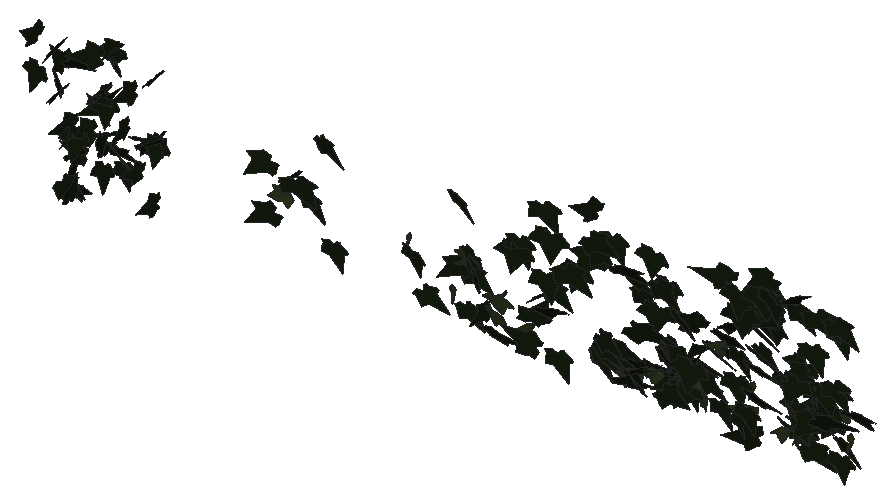
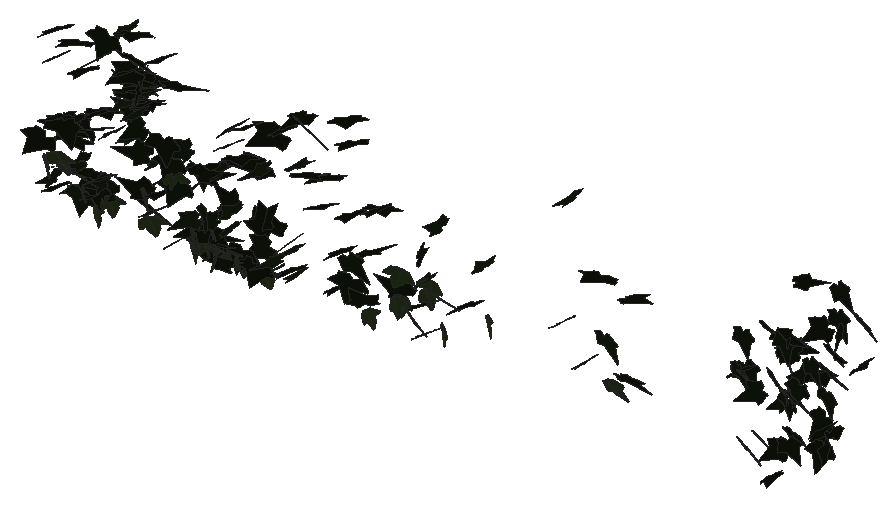
# SketchUp Ruby script. Lengths in millimetres.
U = 1.mm
M = Sketchup.active_model
def pt(a) = Geom::Point3d.new(a.map { |v| v * U })
def face(e, loops, mat)
  f = e.add_face(loops[0].map { |a| pt(a) })
  loops[1..].each { |l| e.add_face(l.map { |a| pt(a) }).erase! }
  f.material = f.back_material = mat if mat
  f
end
# faces: each face lists its corners as indices into pts; further lists are holes
def faces(e, pts, list, mat = nil) = list.each { |f| face(e, (f[0].is_a?(Array) ? f : [f]).map { |l| l.map { |i| pts[i] } }, mat) }
# xy, xz, yz: faces in a plane at the given z, y or x. An outline is a flat list of corners, or four numbers for a rectangle; further outlines are holes
def ring(l) = l.size == 4 ? [[l[0], l[1]], [l[2], l[1]], [l[2], l[3]], [l[0], l[3]]] : l.each_slice(2).to_a
def flat(e, list, mat, &to3) = list.each { |f| face(e, (f[0].is_a?(Array) ? f : [f]).map { |l| ring(l).map { |u, v| to3.(u, v) } }, mat) }
def xy(e, z, list, mat = nil) = flat(e, list, mat) { |x, y| [x, y, z] }
def xz(e, y, list, mat = nil) = flat(e, list, mat) { |x, z| [x, y, z] }
def yz(e, x, list, mat = nil) = flat(e, list, mat) { |y, z| [x, y, z] }
def lines(e, pts, list) = list.each { |a, b| e.add_line(pt(pts[a]), pt(pts[b])) }
# prism: a flat outline (further loops are holes) pulled along v
def prism(e, loops, v, mat = nil)
  f = face(e, loops, mat); d = Geom::Vector3d.new(v.map { |x| x * U })
  f.pushpull(f.normal.samedirection?(d) ? d.length : -d.length)
end
def box(e, o, s, mat = nil) = prism(e, [[o, [o[0] + s[0], o[1], o[2]], [o[0] + s[0], o[1] + s[1], o[2]], [o[0], o[1] + s[1], o[2]]]], [0, 0, s[2]], mat)
def at(x, y, z, deg = 0) = Geom::Transformation.translation(pt([x, y, z])) * Geom::Transformation.rotation(ORIGIN, Z_AXIS, deg.degrees)
def axes(o, x, y, z) = Geom::Transformation.new([*x, 0, *y, 0, *z, 0, *pt(o).to_a, 1])
def part(name) = M.definitions.add(name)
# library, detail: a bought-in or finely detailed component or shape, given as its bounding box
def library(name, o, s) = part(name).tap { |d| box(d.entities, o, s) }
def detail(e, o, s) = box(e.add_group.entities, o, s)
def put(e, d, t, mat = nil) = e.add_instance(d, t).tap { |i| i.material = mat if mat }
def group(e, t, mat = nil) = e.add_group.tap { |g| g.transformation = t; g.material = mat if mat }.entities
root = M.entities
M.materials.add("efeu1").color = [18, 25, 13]
M.materials.add("efeu2").color = [43, 57, 29]
c1 = part("ivyleaf_9")
p = [[39.1,54.8,31.7],[34.5,51.8,30.2],[-5.3,25.2,17.3],[-17.9,28.3,20.9],[-21.6,21.7,17],[-20.2,4.3,5.3],
  [-22.9,-0.3,2.5],[-17.1,-4,-0.6],[-2,-2.1,-1.2],[-0.7,-15.4,-10.1],[16.6,-22.3,-16.7],[21.1,-15.1,-12.5],
  [32.7,-10.7,-11],[46.1,-1.8,-6.6],[30.8,11.2,3.8]]
faces(c1.entities,p,[[0,1,2,3,4,5,6,7,8,9,10,11,12,13,14]],"efeu1")
c2 = part("ivyleaf_10")
p = [[0,12.8,-0.8],[-1.5,51.3,-10.9],[-4.9,51,-11.6],[-13.6,26.5,-7.3],[-13.2,15.9,-4.6],[-21.1,19.3,-7.2],
  [-29.5,16.3,-8.3],[-29.2,8.3,-6.2],[-19.7,-9.8,0.5],[-7.6,-13,4],[1,-12.2,5.8],[-0.4,51.1,-11.1],
  [-1.5,51.1,-10.9],[1,-12.4,5.9],[16.9,-12.4,3.5],[35.1,9.1,-5.1],[35,12.9,-6.1],[20.5,16.4,-4.9],
  [15.8,15,-3.8],[15.3,27.6,-7.1],[12.8,31.3,-7.8]]
faces(c2.entities,p,[[0,1,2,3,4,5,6,7,8,9,10],[11,12,0,13,14,15,16,17,18,19,20]],"efeu2")
put(root,c1,axes([273.7,428,4835.9],[-0.85557,1.08423,0.7221],[-0.62176,0.52637,-1.2853],[-1.46259,-0.858,0.12399]))
put(root,c1,axes([242.2,477.1,4657.7],[-0.36532,-1.32775,0.51119],[-0.11906,-0.50199,-1.36102],[1.73167,-0.31462,0.01427]))
put(root,c1,axes([344.8,510.7,4693.1],[-0.22209,0.63679,1.31638],[-1.04668,1.02774,-0.6158],[-1.44472,-0.84247,0.24378]))
put(root,c1,axes([363.4,626.9,4702.8],[-0.59674,1.20004,-0.36765],[0.22479,-0.32165,-1.29503],[-1.51462,-0.52054,-0.04735]))
put(root,c1,axes([400.9,482.9,4216.3],[-0.00561,-0.17837,1.46528],[0.54141,1.39734,0.1715],[-1.71753,0.44106,0.04927]))
put(root,c1,axes([416.8,537.6,4311.3],[-0.27197,-1.32039,-0.3434],[0.05862,-0.35533,1.33509],[-1.66342,0.20336,0.10319]))
put(root,c1,axes([417.6,371.5,4715.4],[1.01386,-0.28067,-1.21153],[-1.35322,0.49166,-0.87473],[0.68611,1.38445,0.06503]))
put(root,c1,axes([434,676.2,4345.7],[-0.07377,1.1603,-0.56671],[-0.42955,-0.56065,-1.11032],[-1.51569,0.10242,0.34225]))
put(root,c1,axes([444.1,651,4544.6],[-1.33415,0.72884,-0.16345],[0.03182,-0.25235,-1.29979],[-0.91072,-1.07653,0.19402]))
put(root,c1,axes([444.3,349,4884.6],[-0.77185,1.1754,-0.62675],[0.27427,-0.58968,-1.33281],[-1.6018,-0.66735,0.07379]))
put(root,c1,axes([449.2,419.2,4440.2],[-0.37174,1.34751,0.43821],[-0.16281,0.41894,-1.38106],[-1.72103,-0.33069,0.03599]))
put(root,c1,axes([439.7,599.8,4557.9],[0.36998,1.23705,0.48871],[0.02532,0.49679,-1.27039],[-1.62251,0.28984,0.09162]))
put(root,c1,axes([432.2,454,4354.7],[0.66994,1.15124,0.63986],[0.34349,0.57463,-1.27548],[-1.56973,0.61707,-0.00601]))
put(root,c1,axes([425.4,452.9,4758.8],[1.51954,0.5727,0.5016],[0.50025,0.30572,-1.36723],[-0.78257,1.30747,0.09999]))
put(root,c1,axes([444.9,446.4,4213.9],[1.38274,0.72856,-0.4687],[-0.50813,-0.2185,-1.3468],[-0.92673,1.20687,0.03911]))
put(root,c1,axes([489.3,388.7,4527.7],[-1.64876,0.54253,0.34301],[-0.3881,0.12828,-1.45628],[-0.68013,-1.38838,-0.00051]))
put(root,c1,axes([453.5,376.3,4266.3],[0.22516,-0.60274,-1.36473],[-0.17497,1.3616,-0.62075],[1.81169,0.20641,0.10966]))
put(root,c1,axes([495.8,290.9,4720.2],[-0.46741,1.43362,-0.19459],[0.0618,-0.18788,-1.48393],[-1.76397,-0.38646,-0.00043]))
put(root,c1,axes([500.2,620.9,4759.3],[-0.16396,1.3952,-0.04116],[0.01199,-0.04041,-1.40165],[-1.70285,-0.13462,-0.00591]))
put(root,c1,axes([518.3,627.4,4773.2],[-0.26754,-0.15658,-1.36819],[-1.011,-1.09151,0.25774],[-1.34185,0.8536,0.07861]))
put(root,c1,axes([481,720.5,4195.6],[-0.00928,-1.24236,-0.31069],[-0.02096,0.31077,-1.24224],[1.56221,-0.00321,-0.01851]))
put(root,c1,axes([476.1,660.7,4295.4],[1.54093,0.22876,0.34521],[0.41801,0.04508,-1.28351],[-0.28378,1.30861,-0.01613]))
put(root,c1,axes([510.5,630,4681.9],[0.63604,-0.86623,0.94791],[-0.39628,0.90082,1.00185],[-1.51564,-0.59905,0.13585]))
put(root,c1,axes([471.6,540.1,4561],[1.02764,-1.06892,0.55335],[0.42029,-0.43303,-1.36092],[1.40703,0.91005,0.00238]))
put(root,c1,axes([515.7,335.3,4238.7],[-1.21926,0.98729,-0.32059],[-0.33495,0.17776,1.40332],[1.2213,1.03439,0.06482]))
put(root,c1,axes([509.8,391.2,4490.1],[-0.88902,-1.23215,-0.15341],[0.10673,0.12649,-1.43147],[1.51107,-0.73386,0.01085]))
put(root,c1,axes([538.2,445,4496.1],[-0.7733,-0.52593,1.13026],[-0.94644,-0.82614,-0.81947],[1.19053,-0.99837,0.08269]))
put(root,c1,axes([527.9,532.6,4288],[-1.13407,-0.39054,-0.96094],[1.17597,0.15142,-0.99397],[0.46746,-1.32837,0.16922]))
put(root,c1,axes([577.8,501.9,4403.9],[-0.15807,1.16395,0.73041],[-0.26338,0.7073,-1.16542],[-1.65564,-0.22364,0.11566]))
put(root,c1,axes([556.5,471.2,4609.3],[0.39568,0.02009,1.35724],[1.1048,1.03631,-0.23174],[-1.23362,0.93454,0.2278]))
put(root,c1,axes([590.4,461.5,4622.3],[-0.22109,-0.22106,-1.38757],[-0.25021,-1.37992,0.24662],[-1.69582,0.23242,0.14451]))
put(root,c1,axes([606.2,393,4870.9],[-1.02417,-0.18439,1.19989],[-1.38465,-0.39852,-0.85529],[0.52561,-1.40913,0.08488]))
put(root,c1,axes([571.2,448.3,4425.1],[-0.38138,0.87701,1.11033],[0.28619,-1.08925,0.9264],[1.70231,0.3796,0.09301]))
put(root,c1,axes([590.4,468.8,4629.9],[-0.51102,-1.33372,-0.2241],[0.07927,0.21449,-1.39795],[1.64804,-0.42387,-0.00225]))
put(root,c1,axes([577.9,514.2,4410.2],[1.37084,-0.80195,0.15563],[0.15018,-0.09543,-1.38045],[0.98526,1.13034,-0.00613]))
put(root,c1,axes([642.8,610.2,4272],[-1.28412,0.74505,0.34822],[-0.38587,0.15534,-1.28843],[-0.92616,-1.09772,0.05401]))
put(root,c1,axes([639.9,529.9,4511.9],[-1.43164,0.62304,-0.40212],[0.43304,-0.18896,-1.32862],[-0.79429,-1.22599,0.00043]))
put(root,c1,axes([694.9,500.9,4698.8],[-1.57968,0.49729,0.16789],[-0.18829,0.06643,-1.38701],[-0.61203,-1.30396,-0.00663]))
put(root,c1,axes([655.5,574.9,4448],[1.57565,0.15252,0.42652],[0.42907,0.47451,-1.23465],[-0.34826,1.27467,0.40858]))
put(root,c1,axes([702.8,620.3,4710.5],[-0.21174,1.39179,0.02506],[-0.00306,0.02494,-1.40256],[-1.69825,-0.17357,-0.00059]))
put(root,c1,axes([751.8,571.9,4188.3],[-1.51029,0.77954,0.0722],[-0.07438,0.03866,-1.46294],[-0.95221,-1.23944,-0.00023]))
put(root,c1,axes([778.7,516,4492.7],[-0.08106,1.4185,-0.5317],[-0.25474,-0.53571,-1.4031],[-1.83051,0.01173,0.21881]))
put(root,c1,axes([796.7,542.8,4462.4],[-1.30491,0.60869,0.83669],[-0.91036,0.37983,-1.23024],[-0.87444,-1.30377,0.03221]))
put(root,c1,axes([785.8,541.7,4496.2],[-0.6554,1.35212,0.05077],[-0.0876,0.02606,-1.45382],[-1.64843,-0.53898,0.05707]))
put(root,c1,axes([783.9,547.8,4481.5],[-0.55833,-1.36902,0.17153],[0.10373,-0.20836,-1.43612],[1.68007,-0.4421,0.14567]))
put(root,c2,axes([1267.7,738.1,4337.1],[1.34868,-0.41175,-0.9334],[-1.5314,0.47307,-0.81957],[1.19359,1.0722,0.00316]))
put(root,c1,axes([1288.4,631,4313.5],[-2.34815,-0.0339,0.16638],[-0.31584,-0.01743,-1.23419],[0.06836,-1.24484,0.01275]))
put(root,c1,axes([1343.3,535,4603.3],[-1.56454,-0.78213,0.61308],[-0.87792,-0.40443,-1.13447],[1.67525,-0.94238,-0.02196]))
put(root,c1,axes([1359.5,658.4,4477.6],[-0.53506,1.23747,0.10978],[-0.05103,0.10649,-1.269],[-2.36385,-0.2824,0.00255]))
put(root,c1,axes([1402.1,715.4,4382],[0.70204,-1.16725,-0.24276],[-0.05097,0.24593,-1.22322],[2.26848,0.36676,0.04764]))
put(root,c1,axes([1535.1,468.5,4608.6],[-0.5958,-0.87829,-0.93817],[1.31742,0.69832,-0.88473],[2.06074,-0.70037,0.29436]))
put(root,c1,axes([1694.3,504,4363.7],[0.11029,-1.29748,-0.05119],[-0.00218,0.05119,-1.29877],[2.47128,0.05795,0.00114]))
put(root,c1,axes([1709.9,414.3,4874.7],[1.23856,-1.15916,-0.29844],[-0.17967,0.28894,-1.32809],[2.27097,0.65505,0.05769]))
put(root,c2,axes([1908.5,702.4,4378.1],[0.64723,-1.18371,-0.29161],[-0.00315,0.30229,-1.22901],[2.32019,0.33061,0.07968]))
put(root,c1,axes([2086.6,504.3,4469.2],[0.19322,-1.20535,0.54246],[0.18761,-0.53564,-1.20865],[2.50863,0.13289,0.04861]))
put(root,c2,axes([2152.3,675.9,4243.2],[1.0391,-1.09409,-0.25622],[0.18731,0.33033,-1.20082],[2.13038,0.5046,0.23055]))
put(root,c1,axes([2127.5,527.8,4302],[0.86069,-0.89994,-0.83525],[0.00521,0.89084,-0.95835],[2.33677,0.32948,0.30978]))
put(root,c1,axes([2197.1,678.1,4378.7],[-2.3902,0.06796,-0.12555],[0.19895,-0.31928,-1.21851],[-0.18504,-1.22109,0.31161]))
put(root,c2,axes([2214.1,700,4393.8],[-0.79889,-1.18904,0.12701],[-0.03169,-0.12878,-1.26067],[2.27564,-0.41922,0.02703]))
put(root,c2,axes([2214.5,679.5,4422.5],[-2.24534,0.44528,0.13812],[-0.23502,0.06393,-1.2609],[-0.8556,-1.1861,-0.01611]))
put(root,c1,axes([2177.5,660.1,4684.3],[1.08171,-1.14064,0.29714],[0.19719,-0.28026,-1.27401],[2.23463,0.57687,-0.03141]))
put(root,c1,axes([2216.6,701.8,4346.9],[0.62713,-1.03081,-0.64812],[0.27064,0.69941,-1.0401],[2.30154,0.19863,0.29891]))
put(root,c1,axes([2222.4,669.2,4204.3],[0.55168,-1.13046,-0.4308],[0.12869,0.45744,-1.15488],[2.29883,0.24569,0.16804]))
put(root,c1,axes([2240.3,691.9,4425.2],[-0.53139,-0.83368,0.91943],[-0.18544,-0.92478,-0.86812],[2.35481,-0.26096,0.13912]))
put(root,c1,axes([2337.1,656.2,4235],[-1.87063,0.60512,-0.4951],[0.82796,-0.23755,-1.15398],[-1.23641,-1.0746,-0.0237]))
put(root,c2,axes([2373.5,696.4,4296.5],[-0.31496,-1.23971,-0.1588],[0.06072,0.15594,-1.25065],[2.37791,-0.16818,0.0109]))
put(root,c1,axes([2386.9,533.2,4414.8],[-0.14265,-0.80622,1.06803],[0.22519,1.06152,0.80961],[-2.53681,0.13957,0.01181]))
put(root,c2,axes([2400.9,620.9,4259.9],[-2.07147,0.57265,0.29014],[-0.52236,0.10117,-1.22931],[-1.10448,-1.12187,0.03724]))
put(root,c2,axes([2442.8,584.5,4353.1],[-2.39885,0.13065,-0.07539],[0.14357,-0.00345,-1.26717],[-0.24861,-1.26268,-0.00433]))
put(root,c2,axes([2506.3,703.8,4200.5],[-0.33904,-1.20198,0.33615],[-0.00664,-0.33908,-1.21429],[2.37538,-0.17251,0.04458]))
put(root,c1,axes([2462.6,529,4229.3],[0.63332,-0.5275,1.09837],[1.77988,-0.6193,-0.58075],[1.48653,0.96624,0.22741]))
put(root,c1,axes([2525.8,701.9,4240.7],[-1.2335,-0.16836,1.07496],[1.96213,0.30498,0.66936],[-0.66202,1.21761,-0.01902]))
put(root,c1,axes([2524,622.3,4626.8],[-0.05026,-1.34964,-0.23457],[-0.00378,0.23465,-1.34989],[2.60715,-0.02568,-0.00648]))
put(root,c1,axes([2543.1,585.5,4611],[-1.54624,-1.0034,-0.16955],[0.3204,0.08144,-1.28866],[1.91006,-0.82594,0.07891]))
put(root,c1,axes([2612.8,683.8,4398.7],[-0.62784,1.09644,-0.59269],[-0.02164,-0.61572,-1.13272],[-2.37201,-0.2846,0.16721]))
put(root,c1,axes([2592.7,692.8,4313.3],[1.66306,0.90991,-0.20544],[-0.42962,-0.06686,-1.2563],[-1.72257,0.89515,0.11499]))
put(root,c1,axes([2639,683.7,4431.1],[0.53461,-1.07826,-0.65282],[0.04301,0.67304,-1.10192],[2.39856,0.22826,0.16527]))
put(root,c1,axes([2713.8,471.6,4291],[-1.11777,-1.32292,-0.21243],[-0.16078,-0.19492,1.44743],[-2.54495,0.59335,0.00186]))
put(root,c1,axes([2679.7,589.9,4536.1],[-0.35741,-1.33126,-0.24343],[0.01877,0.24441,-1.34423],[2.5756,-0.18652,-0.02398]))
put(root,c1,axes([2675.7,577.2,4850.7],[-0.15353,-1.21087,-0.54346],[0.39536,0.52624,-1.20332],[2.49486,-0.15791,0.15725]))
put(root,c1,axes([2730.5,602.1,4197.8],[0.10072,-1.31287,-0.26727],[-0.0484,0.26644,-1.31386],[2.54944,0.05692,-0.01438]))
put(root,c1,axes([2783,666.7,4566.2],[-1.12944,-1.13866,0.25644],[0.03661,-0.29719,-1.27506],[2.22107,-0.57412,0.15142]))
put(root,c1,axes([2830,435.2,4838.9],[-1.07427,-1.32849,-0.20518],[0.17309,0.18428,-1.44338],[2.55249,-0.57162,0.01152]))
put(root,c1,axes([2891.7,632.2,4879.9],[-1.4527,0.95569,0.57248],[-0.70423,0.43708,-1.223],[-1.99986,-0.84812,0.01482]))
put(root,c1,axes([2820.5,543.7,4634.7],[0.26527,-1.08195,-0.8611],[0.63815,0.86608,-1.03393],[2.55319,-0.10406,0.34789]))
put(root,c1,axes([2874.5,647.8,4668.4],[-1.78407,-0.88542,0.28103],[-0.18224,-0.30503,-1.28042],[1.75856,-0.92987,0.15242]))
put(root,c1,axes([2900.7,655.6,4692.7],[-1.03249,-0.88244,0.8236],[-0.06047,-0.8922,-0.97688],[2.2965,-0.42023,0.34456]))
put(root,c1,axes([2886,662,4224.1],[0.68409,-1.21451,-0.01669],[-0.01492,0.01509,-1.26658],[2.31162,0.35952,-0.00324]))
put(root,c1,axes([2896.7,668.3,4250.4],[0.37727,-1.10014,-0.58465],[0.06465,0.59656,-1.11103],[2.37021,0.15884,0.12336]))
put(root,c1,axes([2936.8,617.4,4344.6],[1.15326,-0.89399,-0.82884],[-0.59063,0.78197,-1.07032],[2.24374,0.66534,0.14427]))
put(root,c1,axes([2930.5,617.9,4301.8],[1.21187,-1.01359,-0.45084],[0.01406,0.52369,-1.16695],[2.11124,0.57832,0.26656]))
put(root,c1,axes([2957.8,695.3,4276.1],[1.81745,-0.67714,-0.50126],[-0.20518,0.65323,-1.08783],[1.59024,0.85818,0.43252]))
put(root,c1,axes([2970.7,515.1,4838.3],[0.45248,-0.63453,-1.24816],[-0.18556,1.25544,-0.65681],[2.65836,0.19564,0.1666]))
put(root,c1,axes([2985.1,693.3,4217.8],[0.17249,-1.2401,0.20466],[0.04842,-0.20334,-1.24337],[2.3916,0.09356,0.01041]))
put(root,c1,axes([2998.5,611.6,4807.5],[-0.05685,-1.31064,-0.22703],[0.09285,0.22586,-1.31027],[2.52985,-0.03774,0.04299]))
put(root,c2,axes([3035.7,693.6,4184.4],[-1.33914,-0.91714,0.50176],[-0.123,-0.56551,-1.12429],[1.98585,-0.65349,0.26872]))
put(root,c1,axes([3042.7,706.9,4227.8],[1.97973,0.55849,-0.37223],[-0.63115,-0.16923,-1.18063],[-1.11055,1.09177,0.00741]))
put(root,c1,axes([3048.1,659,4639.4],[1.86912,-0.69823,-0.53524],[-0.38904,0.59912,-1.15663],[1.62857,0.94448,0.338]))
put(root,c1,axes([3090,593.9,4242.9],[1.22114,0.78271,0.95793],[1.06076,0.78047,-1.01102],[-2.10183,0.84864,0.0463]))
put(root,c1,axes([3076.3,546.1,4730.4],[2.59232,0.27047,0.30087],[0.55735,0.06992,-1.38863],[-0.53125,1.39316,0.01128]))
put(root,c2,axes([3137.9,712.6,4220.9],[-0.01263,-1.25247,-0.04474],[-0.08826,0.04496,-1.25162],[2.38359,-0.00497,-0.04658]))
put(root,c1,axes([3108.6,645.7,4594.9],[0.76758,-1.21333,-0.28459],[-0.03981,0.29249,-1.27665],[2.37154,0.39762,0.07068]))
put(root,c1,axes([3135.5,693.7,4253.6],[1.97846,0.34611,-0.58921],[-1.09315,-0.13857,-1.09476],[-0.70458,1.18685,0.04401]))
put(root,c1,axes([3149,504.9,4259.2],[2.49332,0.3691,0.38071],[-0.6981,-0.10197,1.36107],[0.72879,-1.36045,0.00127]))
put(root,c1,axes([3168.3,653.2,4777.2],[-0.78959,-1.24005,0.23911],[0.04015,-0.25846,-1.30375],[2.4032,-0.40311,0.10034]))
put(root,c2,axes([3139,699.5,4218],[-0.86068,-0.2196,-1.13518],[2.11696,-0.41535,-0.36277],[-0.60066,-1.14918,0.34804]))
put(root,c1,axes([3200.7,500.1,4273.1],[1.08834,-1.10328,0.69756],[-0.5337,0.63994,1.24204],[-2.42624,-0.63566,0.03969]))
put(root,c1,axes([3190.1,692.2,4334],[0.93467,-1.17298,-0.10556],[-0.05157,0.10309,-1.27155],[2.24084,0.49163,0.01477]))
put(root,c1,axes([3259.9,717.7,4169.9],[0.10702,0.11627,1.24014],[-2.06076,0.61816,-0.00886],[-1.17173,-1.07656,0.12885]))
put(root,c1,axes([3207.7,670.4,4388.2],[0.28784,-1.09967,0.65353],[0.39928,-0.62785,-1.10501],[2.40163,0.23618,0.10539]))
put(root,c1,axes([3268.9,699.4,4228.4],[-2.03278,-0.39065,0.51456],[-0.85379,-0.26698,-1.13387],[0.88479,-1.15512,0.08805]))
put(root,c2,axes([3256.3,709,4199.7],[-0.83178,0.90131,0.74431],[-0.65922,0.65909,-1.0015],[-2.12477,-0.55732,0.01934]))
put(root,c1,axes([3200.8,494.5,4526.8],[0.66118,0.07002,-1.38742],[1.56523,1.14223,0.26357],[2.13079,-0.86078,0.2369]))
put(root,c1,axes([3246.9,584.3,4588],[-1.26785,-1.12365,-0.14844],[0.10294,0.14047,-1.30605],[2.15466,-0.66789,-0.02495]))
put(root,c1,axes([3241.3,652.9,4671.5],[-0.28613,-1.30098,0.18184],[0.02771,-0.18467,-1.30916],[2.49993,-0.14686,0.03532]))
put(root,c1,axes([3272.6,707.4,4188.3],[-0.87111,-1.03835,0.5097],[-0.35752,-0.47415,-1.13462],[2.17222,-0.49445,0.01766]))
put(root,c1,axes([3301.8,698.7,4286.1],[-0.0791,0.89421,-0.88564],[-0.65259,-0.86065,-0.85288],[-2.30468,0.21301,0.2719]))
put(root,c2,axes([3289.3,710.9,4231.4],[0.25401,-1.22043,0.23334],[0.23738,-0.22034,-1.22376],[2.35285,0.15399,0.09828]))
put(root,c1,axes([3265.7,562.9,4716.8],[0.85106,-1.16932,-0.66772],[-0.2446,0.66331,-1.24766],[2.55104,0.4537,0.10314]))
put(root,c2,axes([3284.9,687.8,4288.5],[0.4877,-0.69508,1.02635],[0.73268,-0.9516,-0.74058],[2.24249,0.46208,0.01876]))
put(root,c1,axes([3273.3,696.1,4346.8],[1.92725,-0.66498,-0.3712],[-0.45441,0.30923,-1.20532],[1.37635,1.03325,0.12183]))
put(root,c1,axes([3270,663.5,4546.3],[1.0943,-1.16449,0.11352],[0.07065,-0.10826,-1.29863],[2.22565,0.57599,-0.01459]))
put(root,c1,axes([3317.9,704.7,4216.4],[-1.84499,-0.76437,0.22315],[-0.3759,-0.10977,-1.23401],[1.46812,-0.98869,-0.03552]))
put(root,c1,axes([3335.2,643.2,4222.5],[-1.41345,-0.36255,0.93567],[-1.55878,-0.45352,-0.82582],[1.10337,-1.10515,0.03194]))
put(root,c1,axes([3352.5,685.4,4509.7],[-0.19327,-0.01248,1.28198],[-2.43399,0.09101,-0.10042],[-0.1708,-1.28277,-0.0196]))
put(root,c1,axes([3272.4,592.9,4367.8],[0.43639,-0.54167,1.24992],[0.84564,-1.16845,-0.58787],[2.45084,0.49961,-0.01972]))
put(root,c1,axes([3298.9,715.6,4208],[0.15186,-1.23685,0.17262],[0.01058,-0.17262,-1.23941],[2.37676,0.07979,-0.00551]))
put(root,c2,axes([3317.8,707.3,4245.3],[-2.07076,-0.54443,-0.31019],[0.77529,-0.14231,-1.17909],[0.90613,-1.12241,0.29996]))
put(root,c1,axes([3338,662.3,4328.2],[0.10919,0.89717,0.94759],[0.21672,0.94144,-0.89824],[-2.47406,0.12206,-0.03686]))
put(root,c1,axes([3330.9,681.9,4332.6],[-0.77995,-0.96574,0.72072],[-0.26387,-0.71841,-1.04148],[2.27817,-0.41384,0.12611]))
put(root,c2,axes([3355.3,699.1,4296.7],[-0.61311,-1.20135,0.21009],[0.03057,-0.22146,-1.24171],[2.32091,-0.31444,0.07186]))
put(root,c1,axes([3317,698.8,4280.8],[2.3148,-0.12651,0.31625],[0.60186,-0.01626,-1.22272],[0.24084,1.2566,0.01602]))
put(root,c1,axes([3352.8,564.6,4469.2],[-0.45123,-1.17557,0.72144],[-0.27313,-0.70702,-1.19924],[2.61081,-0.27714,-0.00077]))
put(root,c1,axes([3346.8,499.2,4298],[0.69504,-0.60364,-1.26842],[-0.60223,1.24155,-0.68196],[2.60477,0.44812,0.18078]))
put(root,c2,axes([3385.2,693.6,4195.3],[1.27622,-0.88088,-0.61803],[-0.25258,0.65496,-1.07749],[2.03233,0.63455,0.25419]))
put(root,c1,axes([3355.6,712.9,4328],[2.24857,-0.31642,-0.28454],[-0.25593,0.51904,-1.13554],[0.76838,1.09883,0.45445]))
put(root,c1,axes([3432.3,588.3,4458.9],[0.20105,1.06428,0.73257],[-0.27311,0.74013,-1.05458],[-2.44379,0.00484,0.17812]))
put(root,c1,axes([3445.1,700.8,4443.8],[2.13742,0.36716,-0.46141],[-0.96156,0.08737,-1.16021],[-0.57866,1.21101,0.2236]))
put(root,c1,axes([3461.7,519.4,4441.7],[-1.22243,-1.26278,0.00781],[-0.01301,-0.00528,-1.41674],[2.40333,-0.64233,-0.0037]))
put(root,c2,axes([3470.1,700.3,4466.4],[-1.14735,-1.10895,-0.13622],[0.27462,0.07621,-1.25902],[2.10861,-0.61333,0.08985]))
put(root,c1,axes([3455.4,703.3,4189.1],[0.3993,-1.21381,-0.13253],[-0.02805,0.13195,-1.23178],[2.32368,0.21018,0.0079]))
put(root,c1,axes([3473.8,589.4,4361.9],[1.3956,-0.95784,-0.80466],[-0.69238,0.72912,-1.19945],[2.27795,0.80844,0.12841]))
put(root,c1,axes([3497.6,676.6,4521.6],[2.12572,0.20437,-0.61418],[-1.16048,-0.07887,-1.13511],[-0.41343,1.2722,0.0283]))
put(root,c1,axes([3559.1,624.4,4813.8],[-1.30951,0.31455,1.08157],[-2.14255,-0.23406,-0.6481],[0.07107,-1.26033,0.3903]))
put(root,c1,axes([3548.5,670.7,4593],[0.67964,1.22201,-0.28573],[-0.0709,-0.28662,-1.27238],[-2.38741,0.35639,-0.04356]))
put(root,c1,axes([3512.1,566.5,4520.8],[2.17812,-0.58439,-0.19228],[-0.20085,0.2136,-1.2773],[1.15352,1.14066,0.14067]))
put(root,c1,axes([3567.8,668.8,4353.6],[-0.40272,-1.2691,-0.15785],[0.03902,0.15661,-1.28661],[2.43366,-0.21252,-0.00549]))
put(root,c2,axes([3600.7,693.8,4225.3],[-1.48538,-0.88814,0.41455],[-0.20038,-0.45089,-1.16421],[1.85457,-0.76005,0.20624]))
put(root,c1,axes([3584.8,660.7,4477.1],[0.44075,-1.2597,0.25257],[0.11513,-0.24567,-1.28073],[2.44247,0.2389,0.01479]))
put(root,c2,axes([3636.5,683.4,4329.7],[0.75538,-1.14305,-0.37989],[-0.12129,0.37949,-1.20844],[2.28924,0.39728,0.06133]))
put(root,c1,axes([3642.4,620.2,4217.4],[-0.28217,-1.21767,0.33421],[0.14851,-0.3447,-1.22127],[2.39858,-0.12191,0.11493]))
put(root,c1,axes([3654.3,648.4,4711.3],[-0.8152,-1.24571,0.06565],[-0.0351,-0.06308,-1.31729],[2.37387,-0.42872,0.00307]))
put(root,c1,axes([3670.2,641.8,4696.9],[-1.2388,-1.13399,0.15797],[-0.18095,-0.12755,-1.30739],[2.17153,-0.65754,-0.01882]))
put(root,c1,axes([3686.5,648.4,4771.3],[0.41693,-0.20191,-1.28994],[-1.80202,0.87605,-0.29792],[1.711,0.97185,0.00056]))
put(root,c1,axes([3657.6,670.7,4609.4],[2.27116,-0.48176,-0.21472],[-0.37895,0.08036,-1.28691],[0.92956,1.20983,-0.00002]))
put(root,c1,axes([3652.5,642.3,4744.5],[0.87874,-1.23913,0.05503],[0.49722,0.03976,-1.29685],[2.30768,0.46328,0.25847]))
put(root,c1,axes([3663.6,664.2,4674.8],[1.21586,-1.10904,-0.28179],[-0.1161,0.28927,-1.27676],[2.1747,0.6355,0.08939]))
put(root,c1,axes([3706.7,631.5,4741],[-1.70973,-0.86425,0.44533],[-0.41033,-0.41415,-1.23866],[1.8043,-0.91314,0.1403]))
put(root,c1,axes([3745.2,561.3,4204.6],[-2.07806,0.8593,0.50876],[-0.8078,0.28303,-1.38895],[-1.72036,-1.17087,0.03764]))
put(root,c1,axes([3691.6,528.9,4842.8],[-0.65808,-1.39142,0.23096],[-0.04367,-0.23222,-1.43336],[2.68404,-0.34493,0.03331]))
put(root,c1,axes([3655.4,650.4,4313.6],[0.9793,-0.60474,0.99323],[1.52259,-0.60414,-0.78229],[1.60614,0.94143,0.136]))
put(root,c1,axes([3686.8,581.8,4298.6],[0.12644,-1.30132,0.10693],[0.02412,-0.10642,-1.30299],[2.4849,0.06725,0.00721]))
put(root,c1,axes([3707.1,533.7,4761.8],[-1.8419,-0.59131,-0.696],[1.24138,0.26229,-1.1298],[1.2166,-1.16286,0.09908]))
put(root,c1,axes([3742.2,656.8,4723.2],[-2.29613,-0.52985,0.0606],[-0.0602,-0.07853,-1.31635],[1.01319,-1.20542,0.05912]))
put(root,c1,axes([3674.3,627.9,4463.1],[1.65579,-0.61804,0.72556],[1.26723,-0.30878,-1.06143],[1.2979,1.08995,0.11072]))
put(root,c1,axes([3760,635.3,4881.9],[-2.54002,0.10417,-0.0331],[0.04715,-0.10659,-1.3346],[-0.20261,-1.33076,0.1043]))
put(root,c1,axes([3704.3,646.2,4548.8],[1.13815,-1.14853,-0.22201],[-0.05584,0.23454,-1.29235],[2.22564,0.59322,0.08111]))
put(root,c1,axes([3749,611.7,4761.1],[-2.07603,-0.73592,0.0469],[-0.07247,-0.02742,-1.31585],[1.40158,-1.09147,0.00143]))
put(root,c1,axes([3718.5,604.7,4795.7],[-0.26448,-1.01556,-0.92303],[0.19432,0.91753,-1.02487],[2.60462,-0.17158,-0.01727]))
put(root,c1,axes([3759.6,651.7,4737.8],[-1.5934,-0.91955,0.44513],[-0.55016,-0.33876,-1.24351],[1.86488,-0.88562,0.01348]))
put(root,c1,axes([3722.8,636.3,4818.9],[2.50202,0.01191,0.05278],[0.10008,0.02135,-1.31453],[-0.02428,1.31553,0.02085]))
put(root,c1,axes([3745.2,650.3,4821.3],[-0.55329,-1.29724,-0.0253],[0.0263,0.02283,-1.32939],[2.46925,-0.29092,0.00849]))
put(root,c1,axes([3761,663.5,4665],[-0.30435,-1.11113,0.65945],[0.23053,-0.67445,-1.10703],[2.44828,-0.07462,0.18622]))
put(root,c1,axes([3824.8,601.1,4753.1],[-2.2403,0.59332,-0.12824],[0.19259,-0.08409,-1.31787],[-1.13911,-1.1811,0.0294]))
put(root,c2,axes([3823.7,660.1,4223.5],[-0.97978,-1.1581,0.09082],[0.0102,-0.10171,-1.26653],[2.21084,-0.51277,0.04609]))
put(root,c1,axes([3769.1,549.7,4581.3],[0.88888,-0.90512,1.01318],[1.33412,-0.75721,-0.99958],[2.21492,0.81933,0.19548]))
put(root,c1,axes([3832.8,505,4898.4],[-1.20937,-1.12986,-0.38183],[0.59677,0.25915,-1.28867],[2.18996,-0.69456,0.14031]))
put(root,c2,axes([3851.6,705.8,4187.7],[0.22971,-1.20828,-0.25206],[0.12183,0.25905,-1.21113],[2.34595,0.10486,0.08758]))
put(root,c1,axes([3849.8,698.2,4326.1],[-0.78741,-1.13917,0.34819],[-0.1504,-0.34154,-1.21129],[2.26209,-0.41924,0.04067]))
put(root,c1,axes([3828.7,686.3,4313.3],[1.55606,-0.99353,0.04486],[0.05413,-0.03469,-1.28669],[1.89203,0.8181,-0.00008]))
put(root,c1,axes([3819.4,650.8,4250.9],[1.58656,-0.81788,0.58413],[0.75057,-0.43186,-1.16749],[1.75942,0.92176,-0.02869]))
put(root,c1,axes([3856.6,606.3,4488.9],[0.00613,-1.27166,0.22516],[0.08279,-0.22492,-1.27096],[2.45648,0.01075,0.04227]))
put(root,c1,axes([3893.5,666.1,4273],[1.62365,0.19077,-0.95318],[-1.74337,-0.26668,-0.87323],[-0.61919,1.25109,-0.0408]))
put(root,c1,axes([3868.8,506.4,4893.3],[0.09818,-1.35301,0.57577],[0.10574,-0.57392,-1.35364],[2.79651,0.0692,0.03097]))
put(root,c1,axes([3895,687.2,4527.5],[-1.46009,-0.96416,0.37609],[-0.01701,-0.46196,-1.20254],[1.96957,-0.71874,0.26842]))
put(root,c1,axes([3888.1,680.7,4229.3],[-0.1504,-1.21572,-0.26778],[0.06926,0.26594,-1.21815],[2.36821,-0.08499,0.01862]))
put(root,c1,axes([3913,561,4876.4],[1.17624,1.20184,0.31688],[0.24755,0.28941,-1.35134],[-2.35252,0.63136,0.01624]))
put(root,c1,axes([3935.8,696,4229.9],[0.53445,1.17689,0.39667],[0.00967,0.4056,-1.20696],[-2.36365,0.26777,0.08476]))
put(root,c1,axes([3907,618.7,4811.9],[0.69055,-1.20489,-0.44179],[-0.06807,0.44944,-1.25512],[2.44149,0.35332,0.08997]))
put(root,c2,axes([3935.7,679.9,4230.5],[0.65395,-1.10031,0.51908],[0.29619,-0.4952,-1.15271],[2.29642,0.3772,0.00086]))
put(root,c1,axes([3955.2,611.3,4535.4],[-1.21712,-0.52114,1.04747],[-1.10225,-0.8962,-0.79947],[1.93468,-0.83845,0.20349]))
put(root,c1,axes([3956.3,662,4309.1],[-2.04748,-0.66392,0.12963],[-0.19586,-0.08006,-1.2641],[1.27245,-1.08063,0.01401]))
put(root,c1,axes([3962.8,552.8,4530.9],[-1.65928,-0.98057,0.02283],[-0.00418,-0.0286,-1.31199],[1.86673,-0.87166,0.01736]))
put(root,c1,axes([4004.8,711.4,4333.6],[-2.04509,0.55809,0.33362],[-0.71159,-0.00314,-1.19901],[-1.01242,-1.12515,0.16883]))
put(root,c1,axes([3945.1,668.8,4356.7],[1.49069,-1.03521,-0.03],[-0.03232,0.02478,-1.29813],[1.97078,0.78344,0.00141]))
put(root,c1,axes([3960.2,619.4,4486.3],[-0.47159,-0.04645,-1.31287],[2.4442,-0.28978,-0.23213],[-0.52627,-1.30424,0.09833]))
put(root,c1,axes([3983.2,614.3,4218],[0.52777,-0.9616,-0.83083],[0.35611,0.87201,-0.9468],[2.39224,0.08234,0.32424]))
put(root,c2,axes([4050.5,702.6,4358.4],[-2.00298,0.07632,0.6807],[-1.30343,-0.13893,-1.04329],[0.02265,-1.24566,0.15806]))
put(root,c1,axes([4030.1,690,4323],[-1.20189,-0.9735,0.51755],[-0.10738,-0.56712,-1.13558],[2.09557,-0.5874,0.23865]))
put(root,c1,axes([4049.3,631.3,4413.1],[-2.06854,-0.69454,-0.14713],[0.26668,0.05389,-1.28949],[1.3246,-1.09546,0.02985]))
put(root,c1,axes([4026.9,564.4,4695.1],[-0.18218,-1.27306,-0.38239],[0.11951,0.37862,-1.27623],[2.527,-0.10969,0.03279]))
put(root,c1,axes([4065.3,643.5,4480.2],[1.10357,0.98508,-0.65961],[-0.74048,-0.53548,-1.14173],[-2.13131,0.6961,0.05514]))
put(root,c1,axes([4040.3,617.6,4501.3],[-0.5831,-1.19122,-0.49837],[0.2042,0.48694,-1.22988],[2.44904,-0.32422,-0.01611]))
put(root,c1,axes([4027.2,595.2,4831.2],[-0.01472,-1.08691,-0.78547],[0.98071,0.72277,-1.00522],[2.35629,-0.30761,0.41348]))
put(root,c1,axes([4037.2,605,4436.7],[0.82117,-1.20473,-0.0909],[-0.05418,0.08636,-1.27966],[2.29872,0.4324,0.00231]))
put(root,c1,axes([4069.9,644.9,4511.5],[0.03435,-1.16167,-0.58868],[0.01971,0.58884,-1.16168],[2.47848,0.01142,0.0174]))
put(root,c1,axes([4077.3,683.3,4247.2],[1.24591,-1.07935,-0.0328],[-0.02877,0.0292,-1.26236],[2.05496,0.65481,0.00222]))
put(root,c1,axes([4096.4,657.9,4190.4],[-0.35424,-1.25282,0.03415],[-0.02072,-0.03291,-1.26655],[2.38516,-0.18635,-0.00593]))
put(root,c1,axes([4100.7,641.3,4762.3],[0.02213,-1.31954,-0.03233],[0.01229,0.03239,-1.31957],[2.51206,0.01147,0.00674]))
put(root,c1,axes([4084.1,535.5,4409.7],[0.67984,0.50424,-1.15056],[1.27977,0.93362,0.61793],[2.01944,-0.76141,-0.00426]))
put(root,c2,axes([4146.9,656.3,4287.7],[0.93517,-1.12747,-0.26784],[-0.02842,0.28474,-1.226],[2.20534,0.48177,0.09778]))
put(root,c1,axes([4142,670,4398.8],[2.39248,0.30324,-0.10345],[-0.21265,0.02233,-1.29226],[-0.57151,1.26113,0.04776]))
put(root,c1,axes([4141.1,572.3,4844.9],[0.48803,-1.17328,-0.65489],[0.21896,0.68343,-1.17937],[2.54789,0.166,0.22679]))
